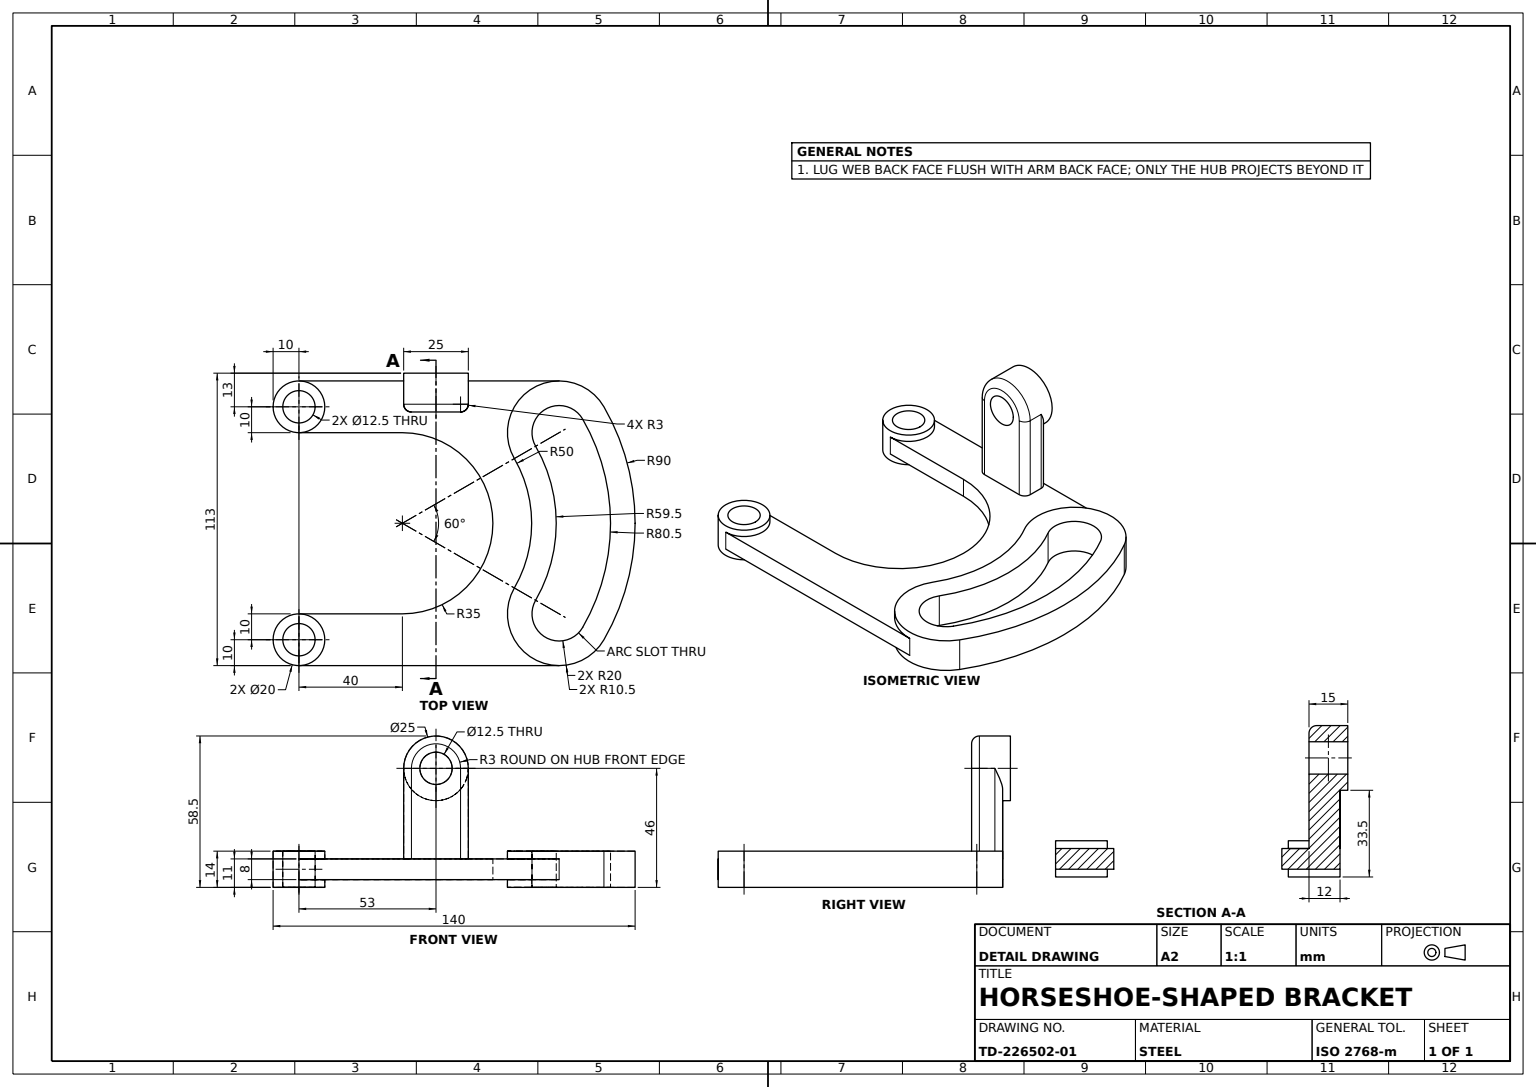
ISO-10303-21;
HEADER;
FILE_DESCRIPTION((''),'2;1');
FILE_NAME('','',(''),(''),'','','');
FILE_SCHEMA(('AUTOMOTIVE_DESIGN'));
ENDSEC;
DATA;
#1=APPLICATION_CONTEXT('');
#2=PRODUCT_CONTEXT('',#1,'mechanical');
#3=PRODUCT('','','',(#2));
#4=PRODUCT_DEFINITION_FORMATION('','',#3);
#5=PRODUCT_DEFINITION_CONTEXT('',#1,'design');
#6=PRODUCT_DEFINITION('','',#4,#5);
#7=PRODUCT_DEFINITION_SHAPE('','',#6);
#8=(LENGTH_UNIT()NAMED_UNIT(*)SI_UNIT(.MILLI.,.METRE.));
#9=(NAMED_UNIT(*)PLANE_ANGLE_UNIT()SI_UNIT($,.RADIAN.));
#10=(NAMED_UNIT(*)SI_UNIT($,.STERADIAN.)SOLID_ANGLE_UNIT());
#11=UNCERTAINTY_MEASURE_WITH_UNIT(LENGTH_MEASURE(1.E-05),#8,'distance_accuracy_value','');
#12=(GEOMETRIC_REPRESENTATION_CONTEXT(3)GLOBAL_UNCERTAINTY_ASSIGNED_CONTEXT((#11))GLOBAL_UNIT_ASSIGNED_CONTEXT((#8,#9,#10))REPRESENTATION_CONTEXT('',''));
#13=CARTESIAN_POINT('',(-43.,39.,-6.75));
#14=VERTEX_POINT('',#13);
#15=CARTESIAN_POINT('',(-58.,39.,-6.75));
#16=VERTEX_POINT('',#15);
#17=CARTESIAN_POINT('',(-25.,39.,-6.75));
#18=DIRECTION('',(-1.,0.,0.));
#19=VECTOR('',#18,1000.);
#20=LINE('',#17,#19);
#21=EDGE_CURVE('',#14,#16,#20,.T.);
#22=ORIENTED_EDGE('',*,*,#21,.T.);
#23=CARTESIAN_POINT('',(-58.,39.,-19.25));
#24=VERTEX_POINT('',#23);
#25=CARTESIAN_POINT('',(-58.,39.,-13.));
#26=DIRECTION('',(0.,0.,1.));
#27=AXIS2_PLACEMENT_3D('',#25,#18,#26);
#28=CIRCLE('',#27,6.25);
#29=EDGE_CURVE('',#16,#24,#28,.T.);
#30=ORIENTED_EDGE('',*,*,#29,.T.);
#31=CARTESIAN_POINT('',(-43.,39.,-19.25));
#32=VERTEX_POINT('',#31);
#33=CARTESIAN_POINT('',(-25.,39.,-19.25));
#34=LINE('',#33,#19);
#35=EDGE_CURVE('',#32,#24,#34,.T.);
#36=ORIENTED_EDGE('',*,*,#35,.F.);
#37=CARTESIAN_POINT('',(-43.,39.,-13.));
#38=AXIS2_PLACEMENT_3D('',#37,#18,#26);
#39=CIRCLE('',#38,6.25);
#40=EDGE_CURVE('',#14,#32,#39,.T.);
#41=ORIENTED_EDGE('',*,*,#40,.F.);
#42=EDGE_LOOP('',(#22,#30,#36,#41));
#43=FACE_OUTER_BOUND('',#42,.T.);
#44=CARTESIAN_POINT('',(-25.,39.,-13.));
#45=AXIS2_PLACEMENT_3D('',#44,#18,#26);
#46=CYLINDRICAL_SURFACE('',#45,6.25);
#47=ADVANCED_FACE('',(#43),#46,.F.);
#48=CARTESIAN_POINT('',(40.25,-7.,-69.715045));
#49=VERTEX_POINT('',#48);
#50=CARTESIAN_POINT('',(0.,-7.,-80.5));
#51=VERTEX_POINT('',#50);
#52=CARTESIAN_POINT('',(0.,-7.,0.));
#53=DIRECTION('',(0.,1.,0.));
#54=AXIS2_PLACEMENT_3D('',#52,#53,#26);
#55=CIRCLE('',#54,80.5);
#56=EDGE_CURVE('',#49,#51,#55,.T.);
#57=ORIENTED_EDGE('',*,*,#56,.T.);
#58=CARTESIAN_POINT('',(-40.25,-7.,-69.715045));
#59=VERTEX_POINT('',#58);
#60=EDGE_CURVE('',#51,#59,#55,.T.);
#61=ORIENTED_EDGE('',*,*,#60,.T.);
#62=CARTESIAN_POINT('',(-29.75,-7.,-51.528512));
#63=VERTEX_POINT('',#62);
#64=CARTESIAN_POINT('',(-35.,-7.,-60.621778));
#65=DIRECTION('',(0.,-1.,0.));
#66=AXIS2_PLACEMENT_3D('',#64,#65,#26);
#67=CIRCLE('',#66,10.5);
#68=EDGE_CURVE('',#63,#59,#67,.T.);
#69=ORIENTED_EDGE('',*,*,#68,.F.);
#70=CARTESIAN_POINT('',(0.,-7.,-59.5));
#71=VERTEX_POINT('',#70);
#72=CIRCLE('',#54,59.5);
#73=EDGE_CURVE('',#71,#63,#72,.T.);
#74=ORIENTED_EDGE('',*,*,#73,.F.);
#75=CARTESIAN_POINT('',(29.75,-7.,-51.528512));
#76=VERTEX_POINT('',#75);
#77=EDGE_CURVE('',#76,#71,#72,.T.);
#78=ORIENTED_EDGE('',*,*,#77,.F.);
#79=CARTESIAN_POINT('',(35.,-7.,-60.621778));
#80=AXIS2_PLACEMENT_3D('',#79,#53,#26);
#81=CIRCLE('',#80,10.5);
#82=EDGE_CURVE('',#76,#49,#81,.T.);
#83=ORIENTED_EDGE('',*,*,#82,.T.);
#84=EDGE_LOOP('',(#57,#61,#69,#74,#78,#83));
#85=FACE_BOUND('',#84,.T.);
#86=CARTESIAN_POINT('',(25.,-7.,-43.30127));
#87=VERTEX_POINT('',#86);
#88=CARTESIAN_POINT('',(0.,-7.,-50.));
#89=VERTEX_POINT('',#88);
#90=CIRCLE('',#54,50.);
#91=EDGE_CURVE('',#87,#89,#90,.T.);
#92=ORIENTED_EDGE('',*,*,#91,.T.);
#93=CARTESIAN_POINT('',(-25.,-7.,-43.30127));
#94=VERTEX_POINT('',#93);
#95=EDGE_CURVE('',#89,#94,#90,.T.);
#96=ORIENTED_EDGE('',*,*,#95,.T.);
#97=CARTESIAN_POINT('',(-45.,-7.,-77.942286));
#98=VERTEX_POINT('',#97);
#99=CIRCLE('',#66,20.);
#100=EDGE_CURVE('',#94,#98,#99,.T.);
#101=ORIENTED_EDGE('',*,*,#100,.T.);
#102=CARTESIAN_POINT('',(0.,-7.,-90.));
#103=VERTEX_POINT('',#102);
#104=CIRCLE('',#54,90.);
#105=EDGE_CURVE('',#103,#98,#104,.T.);
#106=ORIENTED_EDGE('',*,*,#105,.F.);
#107=CARTESIAN_POINT('',(45.,-7.,-77.942286));
#108=VERTEX_POINT('',#107);
#109=EDGE_CURVE('',#108,#103,#104,.T.);
#110=ORIENTED_EDGE('',*,*,#109,.F.);
#111=CIRCLE('',#80,20.);
#112=EDGE_CURVE('',#87,#108,#111,.T.);
#113=ORIENTED_EDGE('',*,*,#112,.F.);
#114=EDGE_LOOP('',(#92,#96,#101,#106,#110,#113));
#115=FACE_OUTER_BOUND('',#114,.T.);
#116=PLANE('',#54);
#117=ADVANCED_FACE('',(#85,#115),#116,.F.);
#118=CARTESIAN_POINT('',(-35.,4.,0.));
#119=VERTEX_POINT('',#118);
#120=CARTESIAN_POINT('',(0.,4.,-35.));
#121=VERTEX_POINT('',#120);
#122=CARTESIAN_POINT('',(0.,4.,0.));
#123=AXIS2_PLACEMENT_3D('',#122,#65,#26);
#124=CIRCLE('',#123,35.);
#125=EDGE_CURVE('',#119,#121,#124,.T.);
#126=ORIENTED_EDGE('',*,*,#125,.F.);
#127=CARTESIAN_POINT('',(-35.,-4.,0.));
#128=VERTEX_POINT('',#127);
#129=VECTOR('',#65,1000.);
#130=LINE('',#118,#129);
#131=EDGE_CURVE('',#119,#128,#130,.T.);
#132=ORIENTED_EDGE('',*,*,#131,.T.);
#133=CARTESIAN_POINT('',(0.,-4.,-35.));
#134=VERTEX_POINT('',#133);
#135=CARTESIAN_POINT('',(0.,-4.,0.));
#136=AXIS2_PLACEMENT_3D('',#135,#65,#26);
#137=CIRCLE('',#136,35.);
#138=EDGE_CURVE('',#128,#134,#137,.T.);
#139=ORIENTED_EDGE('',*,*,#138,.T.);
#140=LINE('',#120,#129);
#141=EDGE_CURVE('',#121,#134,#140,.T.);
#142=ORIENTED_EDGE('',*,*,#141,.F.);
#143=EDGE_LOOP('',(#126,#132,#139,#142));
#144=FACE_OUTER_BOUND('',#143,.T.);
#145=DIRECTION('',(0.,0.,-1.));
#146=AXIS2_PLACEMENT_3D('',#122,#65,#145);
#147=CYLINDRICAL_SURFACE('',#146,35.);
#148=ADVANCED_FACE('',(#144),#147,.F.);
#149=CARTESIAN_POINT('',(-45.,7.,50.));
#150=VERTEX_POINT('',#149);
#151=CARTESIAN_POINT('',(-45.,7.,30.));
#152=VERTEX_POINT('',#151);
#153=CARTESIAN_POINT('',(-45.,7.,40.));
#154=AXIS2_PLACEMENT_3D('',#153,#53,#26);
#155=CIRCLE('',#154,10.);
#156=EDGE_CURVE('',#150,#152,#155,.T.);
#157=ORIENTED_EDGE('',*,*,#156,.T.);
#158=EDGE_CURVE('',#152,#150,#155,.T.);
#159=ORIENTED_EDGE('',*,*,#158,.T.);
#160=EDGE_LOOP('',(#157,#159));
#161=FACE_OUTER_BOUND('',#160,.T.);
#162=CARTESIAN_POINT('',(-45.,7.,33.75));
#163=VERTEX_POINT('',#162);
#164=CARTESIAN_POINT('',(-45.,7.,46.25));
#165=VERTEX_POINT('',#164);
#166=CIRCLE('',#154,6.25);
#167=EDGE_CURVE('',#163,#165,#166,.T.);
#168=ORIENTED_EDGE('',*,*,#167,.F.);
#169=EDGE_CURVE('',#165,#163,#166,.T.);
#170=ORIENTED_EDGE('',*,*,#169,.F.);
#171=EDGE_LOOP('',(#168,#170));
#172=FACE_BOUND('',#171,.T.);
#173=PLANE('',#154);
#174=ADVANCED_FACE('',(#161,#172),#173,.T.);
#175=CARTESIAN_POINT('',(0.,7.,-59.5));
#176=VERTEX_POINT('',#175);
#177=LINE('',#175,#129);
#178=EDGE_CURVE('',#176,#71,#177,.T.);
#179=ORIENTED_EDGE('',*,*,#178,.T.);
#180=ORIENTED_EDGE('',*,*,#73,.T.);
#181=CARTESIAN_POINT('',(-29.75,7.,-51.528512));
#182=VERTEX_POINT('',#181);
#183=LINE('',#181,#129);
#184=EDGE_CURVE('',#182,#63,#183,.T.);
#185=ORIENTED_EDGE('',*,*,#184,.F.);
#186=CARTESIAN_POINT('',(0.,7.,0.));
#187=AXIS2_PLACEMENT_3D('',#186,#53,#26);
#188=CIRCLE('',#187,59.5);
#189=EDGE_CURVE('',#176,#182,#188,.T.);
#190=ORIENTED_EDGE('',*,*,#189,.F.);
#191=EDGE_LOOP('',(#179,#180,#185,#190));
#192=FACE_OUTER_BOUND('',#191,.T.);
#193=AXIS2_PLACEMENT_3D('',#186,#65,#145);
#194=CYLINDRICAL_SURFACE('',#193,59.5);
#195=ADVANCED_FACE('',(#192),#194,.T.);
#196=CARTESIAN_POINT('',(-46.,39.,-25.5));
#197=VERTEX_POINT('',#196);
#198=CARTESIAN_POINT('',(-52.,39.,-25.5));
#199=VERTEX_POINT('',#198);
#200=CARTESIAN_POINT('',(-43.,39.,-25.5));
#201=LINE('',#200,#19);
#202=EDGE_CURVE('',#197,#199,#201,.T.);
#203=ORIENTED_EDGE('',*,*,#202,.T.);
#204=CARTESIAN_POINT('',(-58.,39.,-25.5));
#205=VERTEX_POINT('',#204);
#206=EDGE_CURVE('',#199,#205,#201,.T.);
#207=ORIENTED_EDGE('',*,*,#206,.T.);
#208=CARTESIAN_POINT('',(-58.,39.,-0.5));
#209=VERTEX_POINT('',#208);
#210=CIRCLE('',#27,12.5);
#211=EDGE_CURVE('',#209,#205,#210,.T.);
#212=ORIENTED_EDGE('',*,*,#211,.F.);
#213=CARTESIAN_POINT('',(-52.,39.,-0.5));
#214=VERTEX_POINT('',#213);
#215=CARTESIAN_POINT('',(-43.,39.,-0.5));
#216=LINE('',#215,#19);
#217=EDGE_CURVE('',#214,#209,#216,.T.);
#218=ORIENTED_EDGE('',*,*,#217,.F.);
#219=CARTESIAN_POINT('',(-46.,39.,-0.5));
#220=VERTEX_POINT('',#219);
#221=EDGE_CURVE('',#220,#214,#216,.T.);
#222=ORIENTED_EDGE('',*,*,#221,.F.);
#223=CARTESIAN_POINT('',(-46.,39.,-13.));
#224=AXIS2_PLACEMENT_3D('',#223,#18,#26);
#225=CIRCLE('',#224,12.5);
#226=EDGE_CURVE('',#220,#197,#225,.T.);
#227=ORIENTED_EDGE('',*,*,#226,.T.);
#228=EDGE_LOOP('',(#203,#207,#212,#218,#222,#227));
#229=FACE_OUTER_BOUND('',#228,.T.);
#230=CYLINDRICAL_SURFACE('',#38,12.5);
#231=ADVANCED_FACE('',(#229),#230,.T.);
#232=CARTESIAN_POINT('',(-55.,4.,-3.5));
#233=VERTEX_POINT('',#232);
#234=CARTESIAN_POINT('',(-55.,4.,40.));
#235=VERTEX_POINT('',#234);
#236=CARTESIAN_POINT('',(-55.,4.,-60.621779));
#237=VECTOR('',#26,1000.);
#238=LINE('',#236,#237);
#239=EDGE_CURVE('',#233,#235,#238,.T.);
#240=ORIENTED_EDGE('',*,*,#239,.F.);
#241=CARTESIAN_POINT('',(-55.,30.875962,-3.5));
#242=VERTEX_POINT('',#241);
#243=VECTOR('',#53,1000.);
#244=LINE('',#232,#243);
#245=EDGE_CURVE('',#233,#242,#244,.T.);
#246=ORIENTED_EDGE('',*,*,#245,.T.);
#247=CARTESIAN_POINT('',(-55.,30.875962,-22.5));
#248=VERTEX_POINT('',#247);
#249=CARTESIAN_POINT('',(-55.,39.,-13.));
#250=AXIS2_PLACEMENT_3D('',#249,#18,#26);
#251=CIRCLE('',#250,12.5);
#252=EDGE_CURVE('',#248,#242,#251,.T.);
#253=ORIENTED_EDGE('',*,*,#252,.F.);
#254=CARTESIAN_POINT('',(-55.,4.,-22.5));
#255=VERTEX_POINT('',#254);
#256=LINE('',#254,#129);
#257=EDGE_CURVE('',#248,#255,#256,.T.);
#258=ORIENTED_EDGE('',*,*,#257,.T.);
#259=CARTESIAN_POINT('',(-55.,4.,-60.621778));
#260=VERTEX_POINT('',#259);
#261=EDGE_CURVE('',#260,#255,#238,.T.);
#262=ORIENTED_EDGE('',*,*,#261,.F.);
#263=CARTESIAN_POINT('',(-55.,-4.,-60.621778));
#264=VERTEX_POINT('',#263);
#265=LINE('',#236,#129);
#266=EDGE_CURVE('',#260,#264,#265,.T.);
#267=ORIENTED_EDGE('',*,*,#266,.T.);
#268=CARTESIAN_POINT('',(-55.,-4.,40.));
#269=VERTEX_POINT('',#268);
#270=CARTESIAN_POINT('',(-55.,-4.,-60.621779));
#271=LINE('',#270,#237);
#272=EDGE_CURVE('',#264,#269,#271,.T.);
#273=ORIENTED_EDGE('',*,*,#272,.T.);
#274=LINE('',#234,#129);
#275=EDGE_CURVE('',#235,#269,#274,.T.);
#276=ORIENTED_EDGE('',*,*,#275,.F.);
#277=EDGE_LOOP('',(#240,#246,#253,#258,#262,#267,#273,#276));
#278=FACE_OUTER_BOUND('',#277,.T.);
#279=DIRECTION('',(1.,0.,0.));
#280=AXIS2_PLACEMENT_3D('',#236,#279,#145);
#281=PLANE('',#280);
#282=ADVANCED_FACE('',(#278),#281,.F.);
#283=CARTESIAN_POINT('',(45.,7.,30.));
#284=VERTEX_POINT('',#283);
#285=CARTESIAN_POINT('',(45.,7.,50.));
#286=VERTEX_POINT('',#285);
#287=CARTESIAN_POINT('',(45.,7.,40.));
#288=AXIS2_PLACEMENT_3D('',#287,#53,#26);
#289=CIRCLE('',#288,10.);
#290=EDGE_CURVE('',#284,#286,#289,.T.);
#291=ORIENTED_EDGE('',*,*,#290,.T.);
#292=EDGE_CURVE('',#286,#284,#289,.T.);
#293=ORIENTED_EDGE('',*,*,#292,.T.);
#294=EDGE_LOOP('',(#291,#293));
#295=FACE_OUTER_BOUND('',#294,.T.);
#296=CARTESIAN_POINT('',(45.,7.,33.75));
#297=VERTEX_POINT('',#296);
#298=CARTESIAN_POINT('',(45.,7.,46.25));
#299=VERTEX_POINT('',#298);
#300=CIRCLE('',#288,6.25);
#301=EDGE_CURVE('',#297,#299,#300,.T.);
#302=ORIENTED_EDGE('',*,*,#301,.F.);
#303=EDGE_CURVE('',#299,#297,#300,.T.);
#304=ORIENTED_EDGE('',*,*,#303,.F.);
#305=EDGE_LOOP('',(#302,#304));
#306=FACE_BOUND('',#305,.T.);
#307=PLANE('',#288);
#308=ADVANCED_FACE('',(#295,#306),#307,.T.);
#309=CARTESIAN_POINT('',(0.,-4.,-50.));
#310=VERTEX_POINT('',#309);
#311=CARTESIAN_POINT('',(0.,7.,-50.));
#312=LINE('',#311,#129);
#313=EDGE_CURVE('',#310,#89,#312,.T.);
#314=ORIENTED_EDGE('',*,*,#313,.F.);
#315=CARTESIAN_POINT('',(-25.,-4.,-43.30127));
#316=VERTEX_POINT('',#315);
#317=AXIS2_PLACEMENT_3D('',#135,#53,#26);
#318=CIRCLE('',#317,50.);
#319=EDGE_CURVE('',#310,#316,#318,.T.);
#320=ORIENTED_EDGE('',*,*,#319,.T.);
#321=CARTESIAN_POINT('',(-25.,7.,-43.30127));
#322=LINE('',#321,#129);
#323=EDGE_CURVE('',#316,#94,#322,.T.);
#324=ORIENTED_EDGE('',*,*,#323,.T.);
#325=ORIENTED_EDGE('',*,*,#95,.F.);
#326=EDGE_LOOP('',(#314,#320,#324,#325));
#327=FACE_OUTER_BOUND('',#326,.T.);
#328=CYLINDRICAL_SURFACE('',#193,50.);
#329=ADVANCED_FACE('',(#327),#328,.F.);
#330=CARTESIAN_POINT('',(-45.,-7.,30.));
#331=VERTEX_POINT('',#330);
#332=CARTESIAN_POINT('',(-45.,-7.,50.));
#333=VERTEX_POINT('',#332);
#334=CARTESIAN_POINT('',(-45.,-7.,40.));
#335=AXIS2_PLACEMENT_3D('',#334,#53,#26);
#336=CIRCLE('',#335,10.);
#337=EDGE_CURVE('',#331,#333,#336,.T.);
#338=ORIENTED_EDGE('',*,*,#337,.T.);
#339=LINE('',#332,#243);
#340=EDGE_CURVE('',#333,#150,#339,.T.);
#341=ORIENTED_EDGE('',*,*,#340,.T.);
#342=ORIENTED_EDGE('',*,*,#158,.F.);
#343=CARTESIAN_POINT('',(-45.,4.,30.));
#344=VERTEX_POINT('',#343);
#345=LINE('',#330,#243);
#346=EDGE_CURVE('',#344,#152,#345,.T.);
#347=ORIENTED_EDGE('',*,*,#346,.F.);
#348=CARTESIAN_POINT('',(-45.,4.,40.));
#349=AXIS2_PLACEMENT_3D('',#348,#65,#145);
#350=CIRCLE('',#349,10.);
#351=EDGE_CURVE('',#235,#344,#350,.T.);
#352=ORIENTED_EDGE('',*,*,#351,.F.);
#353=ORIENTED_EDGE('',*,*,#275,.T.);
#354=CARTESIAN_POINT('',(-45.,-4.,30.));
#355=VERTEX_POINT('',#354);
#356=CARTESIAN_POINT('',(-45.,-4.,40.));
#357=AXIS2_PLACEMENT_3D('',#356,#65,#145);
#358=CIRCLE('',#357,10.);
#359=EDGE_CURVE('',#269,#355,#358,.T.);
#360=ORIENTED_EDGE('',*,*,#359,.T.);
#361=EDGE_CURVE('',#331,#355,#345,.T.);
#362=ORIENTED_EDGE('',*,*,#361,.F.);
#363=EDGE_LOOP('',(#338,#341,#342,#347,#352,#353,#360,#362));
#364=FACE_OUTER_BOUND('',#363,.T.);
#365=CYLINDRICAL_SURFACE('',#335,10.);
#366=ADVANCED_FACE('',(#364),#365,.T.);
#367=ORIENTED_EDGE('',*,*,#77,.T.);
#368=ORIENTED_EDGE('',*,*,#178,.F.);
#369=CARTESIAN_POINT('',(29.75,7.,-51.528512));
#370=VERTEX_POINT('',#369);
#371=EDGE_CURVE('',#370,#176,#188,.T.);
#372=ORIENTED_EDGE('',*,*,#371,.F.);
#373=LINE('',#369,#129);
#374=EDGE_CURVE('',#370,#76,#373,.T.);
#375=ORIENTED_EDGE('',*,*,#374,.T.);
#376=EDGE_LOOP('',(#367,#368,#372,#375));
#377=FACE_OUTER_BOUND('',#376,.T.);
#378=ADVANCED_FACE('',(#377),#194,.T.);
#379=CARTESIAN_POINT('',(35.,4.,0.));
#380=VERTEX_POINT('',#379);
#381=CARTESIAN_POINT('',(35.,4.,40.));
#382=VERTEX_POINT('',#381);
#383=LINE('',#379,#237);
#384=EDGE_CURVE('',#380,#382,#383,.T.);
#385=ORIENTED_EDGE('',*,*,#384,.F.);
#386=CARTESIAN_POINT('',(35.,-4.,0.));
#387=VERTEX_POINT('',#386);
#388=LINE('',#379,#129);
#389=EDGE_CURVE('',#380,#387,#388,.T.);
#390=ORIENTED_EDGE('',*,*,#389,.T.);
#391=CARTESIAN_POINT('',(35.,-4.,40.));
#392=VERTEX_POINT('',#391);
#393=LINE('',#386,#237);
#394=EDGE_CURVE('',#387,#392,#393,.T.);
#395=ORIENTED_EDGE('',*,*,#394,.T.);
#396=LINE('',#381,#129);
#397=EDGE_CURVE('',#382,#392,#396,.T.);
#398=ORIENTED_EDGE('',*,*,#397,.F.);
#399=EDGE_LOOP('',(#385,#390,#395,#398));
#400=FACE_OUTER_BOUND('',#399,.T.);
#401=AXIS2_PLACEMENT_3D('',#379,#279,#145);
#402=PLANE('',#401);
#403=ADVANCED_FACE('',(#400),#402,.F.);
#404=CARTESIAN_POINT('',(-35.,-4.,-60.621779));
#405=AXIS2_PLACEMENT_3D('',#404,#65,#26);
#406=CIRCLE('',#405,20.);
#407=EDGE_CURVE('',#316,#264,#406,.T.);
#408=ORIENTED_EDGE('',*,*,#407,.T.);
#409=ORIENTED_EDGE('',*,*,#266,.F.);
#410=CARTESIAN_POINT('',(-25.,4.,-43.30127));
#411=VERTEX_POINT('',#410);
#412=CARTESIAN_POINT('',(-35.,4.,-60.621779));
#413=AXIS2_PLACEMENT_3D('',#412,#65,#26);
#414=CIRCLE('',#413,20.);
#415=EDGE_CURVE('',#411,#260,#414,.T.);
#416=ORIENTED_EDGE('',*,*,#415,.F.);
#417=VERTEX_POINT('',#321);
#418=EDGE_CURVE('',#417,#411,#322,.T.);
#419=ORIENTED_EDGE('',*,*,#418,.F.);
#420=CARTESIAN_POINT('',(-45.,7.,-77.942286));
#421=VERTEX_POINT('',#420);
#422=CARTESIAN_POINT('',(-35.,7.,-60.621778));
#423=AXIS2_PLACEMENT_3D('',#422,#65,#26);
#424=CIRCLE('',#423,20.);
#425=EDGE_CURVE('',#417,#421,#424,.T.);
#426=ORIENTED_EDGE('',*,*,#425,.T.);
#427=LINE('',#420,#129);
#428=EDGE_CURVE('',#421,#98,#427,.T.);
#429=ORIENTED_EDGE('',*,*,#428,.T.);
#430=ORIENTED_EDGE('',*,*,#100,.F.);
#431=ORIENTED_EDGE('',*,*,#323,.F.);
#432=EDGE_LOOP('',(#408,#409,#416,#419,#426,#429,#430,#431));
#433=FACE_OUTER_BOUND('',#432,.T.);
#434=AXIS2_PLACEMENT_3D('',#422,#65,#145);
#435=CYLINDRICAL_SURFACE('',#434,20.);
#436=ADVANCED_FACE('',(#433),#435,.T.);
#437=CARTESIAN_POINT('',(-46.,4.,-25.5));
#438=VERTEX_POINT('',#437);
#439=CARTESIAN_POINT('',(-52.,4.,-25.5));
#440=VERTEX_POINT('',#439);
#441=CARTESIAN_POINT('',(-43.,4.,-25.5));
#442=LINE('',#441,#19);
#443=EDGE_CURVE('',#438,#440,#442,.T.);
#444=ORIENTED_EDGE('',*,*,#443,.T.);
#445=LINE('',#198,#243);
#446=EDGE_CURVE('',#440,#199,#445,.T.);
#447=ORIENTED_EDGE('',*,*,#446,.T.);
#448=ORIENTED_EDGE('',*,*,#202,.F.);
#449=LINE('',#437,#129);
#450=EDGE_CURVE('',#197,#438,#449,.T.);
#451=ORIENTED_EDGE('',*,*,#450,.T.);
#452=EDGE_LOOP('',(#444,#447,#448,#451));
#453=FACE_OUTER_BOUND('',#452,.T.);
#454=CARTESIAN_POINT('',(-43.,0.,-25.5));
#455=AXIS2_PLACEMENT_3D('',#454,#145,#18);
#456=PLANE('',#455);
#457=ADVANCED_FACE('',(#453),#456,.T.);
#458=EDGE_CURVE('',#205,#209,#210,.T.);
#459=ORIENTED_EDGE('',*,*,#458,.T.);
#460=ORIENTED_EDGE('',*,*,#211,.T.);
#461=EDGE_LOOP('',(#459,#460));
#462=FACE_OUTER_BOUND('',#461,.T.);
#463=ORIENTED_EDGE('',*,*,#29,.F.);
#464=EDGE_CURVE('',#24,#16,#28,.T.);
#465=ORIENTED_EDGE('',*,*,#464,.F.);
#466=EDGE_LOOP('',(#463,#465));
#467=FACE_BOUND('',#466,.T.);
#468=PLANE('',#27);
#469=ADVANCED_FACE('',(#462,#467),#468,.T.);
#470=ORIENTED_EDGE('',*,*,#389,.F.);
#471=EDGE_CURVE('',#121,#380,#124,.T.);
#472=ORIENTED_EDGE('',*,*,#471,.F.);
#473=ORIENTED_EDGE('',*,*,#141,.T.);
#474=EDGE_CURVE('',#134,#387,#137,.T.);
#475=ORIENTED_EDGE('',*,*,#474,.T.);
#476=EDGE_LOOP('',(#470,#472,#473,#475));
#477=FACE_OUTER_BOUND('',#476,.T.);
#478=ADVANCED_FACE('',(#477),#147,.F.);
#479=ORIENTED_EDGE('',*,*,#91,.F.);
#480=CARTESIAN_POINT('',(25.,-4.,-43.30127));
#481=VERTEX_POINT('',#480);
#482=CARTESIAN_POINT('',(25.,7.,-43.30127));
#483=LINE('',#482,#129);
#484=EDGE_CURVE('',#481,#87,#483,.T.);
#485=ORIENTED_EDGE('',*,*,#484,.F.);
#486=EDGE_CURVE('',#481,#310,#318,.T.);
#487=ORIENTED_EDGE('',*,*,#486,.T.);
#488=ORIENTED_EDGE('',*,*,#313,.T.);
#489=EDGE_LOOP('',(#479,#485,#487,#488));
#490=FACE_OUTER_BOUND('',#489,.T.);
#491=ADVANCED_FACE('',(#490),#328,.F.);
#492=CARTESIAN_POINT('',(-45.,-7.,46.25));
#493=VERTEX_POINT('',#492);
#494=CARTESIAN_POINT('',(-45.,-38.,46.25));
#495=LINE('',#494,#243);
#496=EDGE_CURVE('',#493,#165,#495,.T.);
#497=ORIENTED_EDGE('',*,*,#496,.T.);
#498=ORIENTED_EDGE('',*,*,#169,.T.);
#499=CARTESIAN_POINT('',(-45.,-7.,33.75));
#500=VERTEX_POINT('',#499);
#501=CARTESIAN_POINT('',(-45.,-38.,33.75));
#502=LINE('',#501,#243);
#503=EDGE_CURVE('',#500,#163,#502,.T.);
#504=ORIENTED_EDGE('',*,*,#503,.F.);
#505=CIRCLE('',#335,6.25);
#506=EDGE_CURVE('',#493,#500,#505,.T.);
#507=ORIENTED_EDGE('',*,*,#506,.F.);
#508=EDGE_LOOP('',(#497,#498,#504,#507));
#509=FACE_OUTER_BOUND('',#508,.T.);
#510=CARTESIAN_POINT('',(-45.,-38.,40.));
#511=AXIS2_PLACEMENT_3D('',#510,#53,#26);
#512=CYLINDRICAL_SURFACE('',#511,6.25);
#513=ADVANCED_FACE('',(#509),#512,.F.);
#514=ORIENTED_EDGE('',*,*,#167,.T.);
#515=ORIENTED_EDGE('',*,*,#496,.F.);
#516=EDGE_CURVE('',#500,#493,#505,.T.);
#517=ORIENTED_EDGE('',*,*,#516,.F.);
#518=ORIENTED_EDGE('',*,*,#503,.T.);
#519=EDGE_LOOP('',(#514,#515,#517,#518));
#520=FACE_OUTER_BOUND('',#519,.T.);
#521=ADVANCED_FACE('',(#520),#512,.F.);
#522=EDGE_CURVE('',#32,#14,#39,.T.);
#523=ORIENTED_EDGE('',*,*,#522,.F.);
#524=ORIENTED_EDGE('',*,*,#35,.T.);
#525=ORIENTED_EDGE('',*,*,#464,.T.);
#526=ORIENTED_EDGE('',*,*,#21,.F.);
#527=EDGE_LOOP('',(#523,#524,#525,#526));
#528=FACE_OUTER_BOUND('',#527,.T.);
#529=ADVANCED_FACE('',(#528),#46,.F.);
#530=CARTESIAN_POINT('',(-43.,39.,-22.5));
#531=VERTEX_POINT('',#530);
#532=CARTESIAN_POINT('',(-46.,39.,-22.5));
#533=AXIS2_PLACEMENT_3D('',#532,#65,#145);
#534=CIRCLE('',#533,3.);
#535=EDGE_CURVE('',#197,#531,#534,.T.);
#536=ORIENTED_EDGE('',*,*,#535,.F.);
#537=ORIENTED_EDGE('',*,*,#226,.F.);
#538=CARTESIAN_POINT('',(-43.,39.,-3.5));
#539=VERTEX_POINT('',#538);
#540=CARTESIAN_POINT('',(-46.,39.,-3.5));
#541=AXIS2_PLACEMENT_3D('',#540,#53,#26);
#542=CIRCLE('',#541,3.);
#543=EDGE_CURVE('',#220,#539,#542,.T.);
#544=ORIENTED_EDGE('',*,*,#543,.T.);
#545=AXIS2_PLACEMENT_3D('',#37,#279,#26);
#546=CIRCLE('',#545,9.5);
#547=EDGE_CURVE('',#531,#539,#546,.T.);
#548=ORIENTED_EDGE('',*,*,#547,.F.);
#549=EDGE_LOOP('',(#536,#537,#544,#548));
#550=FACE_OUTER_BOUND('',#549,.T.);
#551=TOROIDAL_SURFACE('',#224,9.5,3.);
#552=ADVANCED_FACE('',(#550),#551,.T.);
#553=CARTESIAN_POINT('',(55.,-4.,40.));
#554=VERTEX_POINT('',#553);
#555=CARTESIAN_POINT('',(55.,-4.,-60.621779));
#556=VERTEX_POINT('',#555);
#557=VECTOR('',#145,1000.);
#558=LINE('',#555,#557);
#559=EDGE_CURVE('',#554,#556,#558,.T.);
#560=ORIENTED_EDGE('',*,*,#559,.T.);
#561=CARTESIAN_POINT('',(55.,4.,-60.621778));
#562=VERTEX_POINT('',#561);
#563=CARTESIAN_POINT('',(55.,4.,-60.621779));
#564=LINE('',#563,#129);
#565=EDGE_CURVE('',#562,#556,#564,.T.);
#566=ORIENTED_EDGE('',*,*,#565,.F.);
#567=CARTESIAN_POINT('',(55.,4.,40.));
#568=VERTEX_POINT('',#567);
#569=LINE('',#567,#557);
#570=EDGE_CURVE('',#568,#562,#569,.T.);
#571=ORIENTED_EDGE('',*,*,#570,.F.);
#572=LINE('',#567,#129);
#573=EDGE_CURVE('',#568,#554,#572,.T.);
#574=ORIENTED_EDGE('',*,*,#573,.T.);
#575=EDGE_LOOP('',(#560,#566,#571,#574));
#576=FACE_OUTER_BOUND('',#575,.T.);
#577=AXIS2_PLACEMENT_3D('',#563,#18,#26);
#578=PLANE('',#577);
#579=ADVANCED_FACE('',(#576),#578,.F.);
#580=ORIENTED_EDGE('',*,*,#397,.T.);
#581=CARTESIAN_POINT('',(45.,-4.,30.));
#582=VERTEX_POINT('',#581);
#583=CARTESIAN_POINT('',(45.,-4.,40.));
#584=AXIS2_PLACEMENT_3D('',#583,#65,#145);
#585=CIRCLE('',#584,10.);
#586=EDGE_CURVE('',#392,#582,#585,.T.);
#587=ORIENTED_EDGE('',*,*,#586,.T.);
#588=CARTESIAN_POINT('',(45.,-7.,30.));
#589=VERTEX_POINT('',#588);
#590=LINE('',#588,#243);
#591=EDGE_CURVE('',#589,#582,#590,.T.);
#592=ORIENTED_EDGE('',*,*,#591,.F.);
#593=CARTESIAN_POINT('',(45.,-7.,50.));
#594=VERTEX_POINT('',#593);
#595=CARTESIAN_POINT('',(45.,-7.,40.));
#596=AXIS2_PLACEMENT_3D('',#595,#53,#26);
#597=CIRCLE('',#596,10.);
#598=EDGE_CURVE('',#589,#594,#597,.T.);
#599=ORIENTED_EDGE('',*,*,#598,.T.);
#600=LINE('',#593,#243);
#601=EDGE_CURVE('',#594,#286,#600,.T.);
#602=ORIENTED_EDGE('',*,*,#601,.T.);
#603=ORIENTED_EDGE('',*,*,#290,.F.);
#604=CARTESIAN_POINT('',(45.,4.,30.));
#605=VERTEX_POINT('',#604);
#606=EDGE_CURVE('',#605,#284,#590,.T.);
#607=ORIENTED_EDGE('',*,*,#606,.F.);
#608=CARTESIAN_POINT('',(45.,4.,40.));
#609=AXIS2_PLACEMENT_3D('',#608,#65,#145);
#610=CIRCLE('',#609,10.);
#611=EDGE_CURVE('',#382,#605,#610,.T.);
#612=ORIENTED_EDGE('',*,*,#611,.F.);
#613=EDGE_LOOP('',(#580,#587,#592,#599,#602,#603,#607,#612));
#614=FACE_OUTER_BOUND('',#613,.T.);
#615=CYLINDRICAL_SURFACE('',#596,10.);
#616=ADVANCED_FACE('',(#614),#615,.T.);
#617=CARTESIAN_POINT('',(25.,4.,-43.30127));
#618=VERTEX_POINT('',#617);
#619=CARTESIAN_POINT('',(0.,4.,-50.));
#620=VERTEX_POINT('',#619);
#621=AXIS2_PLACEMENT_3D('',#122,#53,#26);
#622=CIRCLE('',#621,50.);
#623=EDGE_CURVE('',#618,#620,#622,.T.);
#624=ORIENTED_EDGE('',*,*,#623,.T.);
#625=EDGE_CURVE('',#620,#411,#622,.T.);
#626=ORIENTED_EDGE('',*,*,#625,.T.);
#627=ORIENTED_EDGE('',*,*,#415,.T.);
#628=ORIENTED_EDGE('',*,*,#261,.T.);
#629=CARTESIAN_POINT('',(-52.,4.,-22.5));
#630=AXIS2_PLACEMENT_3D('',#629,#65,#145);
#631=CIRCLE('',#630,3.);
#632=EDGE_CURVE('',#255,#440,#631,.T.);
#633=ORIENTED_EDGE('',*,*,#632,.T.);
#634=ORIENTED_EDGE('',*,*,#443,.F.);
#635=CARTESIAN_POINT('',(-43.,4.,-22.5));
#636=VERTEX_POINT('',#635);
#637=CARTESIAN_POINT('',(-46.,4.,-22.5));
#638=AXIS2_PLACEMENT_3D('',#637,#65,#145);
#639=CIRCLE('',#638,3.);
#640=EDGE_CURVE('',#438,#636,#639,.T.);
#641=ORIENTED_EDGE('',*,*,#640,.T.);
#642=CARTESIAN_POINT('',(-43.,4.,-3.5));
#643=VERTEX_POINT('',#642);
#644=CARTESIAN_POINT('',(-43.,4.,0.));
#645=LINE('',#644,#557);
#646=EDGE_CURVE('',#643,#636,#645,.T.);
#647=ORIENTED_EDGE('',*,*,#646,.F.);
#648=CARTESIAN_POINT('',(-46.,4.,-0.5));
#649=VERTEX_POINT('',#648);
#650=CARTESIAN_POINT('',(-46.,4.,-3.5));
#651=AXIS2_PLACEMENT_3D('',#650,#65,#145);
#652=CIRCLE('',#651,3.);
#653=EDGE_CURVE('',#643,#649,#652,.T.);
#654=ORIENTED_EDGE('',*,*,#653,.T.);
#655=CARTESIAN_POINT('',(-52.,4.,-0.5));
#656=VERTEX_POINT('',#655);
#657=CARTESIAN_POINT('',(-43.,4.,-0.5));
#658=LINE('',#657,#19);
#659=EDGE_CURVE('',#649,#656,#658,.T.);
#660=ORIENTED_EDGE('',*,*,#659,.T.);
#661=CARTESIAN_POINT('',(-52.,4.,-3.5));
#662=AXIS2_PLACEMENT_3D('',#661,#65,#145);
#663=CIRCLE('',#662,3.);
#664=EDGE_CURVE('',#656,#233,#663,.T.);
#665=ORIENTED_EDGE('',*,*,#664,.T.);
#666=ORIENTED_EDGE('',*,*,#239,.T.);
#667=ORIENTED_EDGE('',*,*,#351,.T.);
#668=CARTESIAN_POINT('',(-35.,4.,40.));
#669=VERTEX_POINT('',#668);
#670=EDGE_CURVE('',#344,#669,#350,.T.);
#671=ORIENTED_EDGE('',*,*,#670,.T.);
#672=LINE('',#118,#557);
#673=EDGE_CURVE('',#669,#119,#672,.T.);
#674=ORIENTED_EDGE('',*,*,#673,.T.);
#675=ORIENTED_EDGE('',*,*,#125,.T.);
#676=ORIENTED_EDGE('',*,*,#471,.T.);
#677=ORIENTED_EDGE('',*,*,#384,.T.);
#678=ORIENTED_EDGE('',*,*,#611,.T.);
#679=EDGE_CURVE('',#605,#568,#610,.T.);
#680=ORIENTED_EDGE('',*,*,#679,.T.);
#681=ORIENTED_EDGE('',*,*,#570,.T.);
#682=CARTESIAN_POINT('',(35.,4.,-60.621779));
#683=AXIS2_PLACEMENT_3D('',#682,#65,#145);
#684=CIRCLE('',#683,20.);
#685=EDGE_CURVE('',#562,#618,#684,.T.);
#686=ORIENTED_EDGE('',*,*,#685,.T.);
#687=EDGE_LOOP('',(#624,#626,#627,#628,#633,#634,#641,#647,#654,#660,#665,#666,#667,#671,#674,#675,#676,#677,#678,#680,#681,#686));
#688=FACE_OUTER_BOUND('',#687,.T.);
#689=PLANE('',#683);
#690=ADVANCED_FACE('',(#688),#689,.F.);
#691=CARTESIAN_POINT('',(40.25,7.,-69.715045));
#692=VERTEX_POINT('',#691);
#693=CARTESIAN_POINT('',(35.,7.,-60.621778));
#694=AXIS2_PLACEMENT_3D('',#693,#53,#26);
#695=CIRCLE('',#694,10.5);
#696=EDGE_CURVE('',#370,#692,#695,.T.);
#697=ORIENTED_EDGE('',*,*,#696,.T.);
#698=LINE('',#691,#129);
#699=EDGE_CURVE('',#692,#49,#698,.T.);
#700=ORIENTED_EDGE('',*,*,#699,.T.);
#701=ORIENTED_EDGE('',*,*,#82,.F.);
#702=ORIENTED_EDGE('',*,*,#374,.F.);
#703=EDGE_LOOP('',(#697,#700,#701,#702));
#704=FACE_OUTER_BOUND('',#703,.T.);
#705=AXIS2_PLACEMENT_3D('',#693,#65,#145);
#706=CYLINDRICAL_SURFACE('',#705,10.5);
#707=ADVANCED_FACE('',(#704),#706,.F.);
#708=CARTESIAN_POINT('',(0.,7.,-80.5));
#709=VERTEX_POINT('',#708);
#710=LINE('',#708,#129);
#711=EDGE_CURVE('',#709,#51,#710,.T.);
#712=ORIENTED_EDGE('',*,*,#711,.F.);
#713=CARTESIAN_POINT('',(-40.25,7.,-69.715045));
#714=VERTEX_POINT('',#713);
#715=CIRCLE('',#187,80.5);
#716=EDGE_CURVE('',#709,#714,#715,.T.);
#717=ORIENTED_EDGE('',*,*,#716,.T.);
#718=LINE('',#713,#129);
#719=EDGE_CURVE('',#714,#59,#718,.T.);
#720=ORIENTED_EDGE('',*,*,#719,.T.);
#721=ORIENTED_EDGE('',*,*,#60,.F.);
#722=EDGE_LOOP('',(#712,#717,#720,#721));
#723=FACE_OUTER_BOUND('',#722,.T.);
#724=CYLINDRICAL_SURFACE('',#193,80.5);
#725=ADVANCED_FACE('',(#723),#724,.F.);
#726=ORIENTED_EDGE('',*,*,#105,.T.);
#727=ORIENTED_EDGE('',*,*,#428,.F.);
#728=CARTESIAN_POINT('',(0.,7.,-90.));
#729=VERTEX_POINT('',#728);
#730=CIRCLE('',#187,90.);
#731=EDGE_CURVE('',#729,#421,#730,.T.);
#732=ORIENTED_EDGE('',*,*,#731,.F.);
#733=LINE('',#728,#129);
#734=EDGE_CURVE('',#729,#103,#733,.T.);
#735=ORIENTED_EDGE('',*,*,#734,.T.);
#736=EDGE_LOOP('',(#726,#727,#732,#735));
#737=FACE_OUTER_BOUND('',#736,.T.);
#738=CYLINDRICAL_SURFACE('',#193,90.);
#739=ADVANCED_FACE('',(#737),#738,.T.);
#740=ORIENTED_EDGE('',*,*,#659,.F.);
#741=CARTESIAN_POINT('',(-46.,0.,-0.5));
#742=LINE('',#741,#243);
#743=EDGE_CURVE('',#649,#220,#742,.T.);
#744=ORIENTED_EDGE('',*,*,#743,.T.);
#745=ORIENTED_EDGE('',*,*,#221,.T.);
#746=CARTESIAN_POINT('',(-52.,0.,-0.5));
#747=LINE('',#746,#129);
#748=EDGE_CURVE('',#214,#656,#747,.T.);
#749=ORIENTED_EDGE('',*,*,#748,.T.);
#750=EDGE_LOOP('',(#740,#744,#745,#749));
#751=FACE_OUTER_BOUND('',#750,.T.);
#752=CARTESIAN_POINT('',(-43.,0.,-0.5));
#753=AXIS2_PLACEMENT_3D('',#752,#145,#18);
#754=PLANE('',#753);
#755=ADVANCED_FACE('',(#751),#754,.F.);
#756=EDGE_CURVE('',#333,#331,#336,.T.);
#757=ORIENTED_EDGE('',*,*,#756,.F.);
#758=ORIENTED_EDGE('',*,*,#337,.F.);
#759=EDGE_LOOP('',(#757,#758));
#760=FACE_OUTER_BOUND('',#759,.T.);
#761=ORIENTED_EDGE('',*,*,#506,.T.);
#762=ORIENTED_EDGE('',*,*,#516,.T.);
#763=EDGE_LOOP('',(#761,#762));
#764=FACE_BOUND('',#763,.T.);
#765=PLANE('',#335);
#766=ADVANCED_FACE('',(#760,#764),#765,.F.);
#767=ORIENTED_EDGE('',*,*,#586,.F.);
#768=ORIENTED_EDGE('',*,*,#394,.F.);
#769=ORIENTED_EDGE('',*,*,#474,.F.);
#770=ORIENTED_EDGE('',*,*,#138,.F.);
#771=CARTESIAN_POINT('',(-35.,-4.,40.));
#772=VERTEX_POINT('',#771);
#773=LINE('',#127,#557);
#774=EDGE_CURVE('',#772,#128,#773,.T.);
#775=ORIENTED_EDGE('',*,*,#774,.F.);
#776=EDGE_CURVE('',#355,#772,#358,.T.);
#777=ORIENTED_EDGE('',*,*,#776,.F.);
#778=ORIENTED_EDGE('',*,*,#359,.F.);
#779=ORIENTED_EDGE('',*,*,#272,.F.);
#780=ORIENTED_EDGE('',*,*,#407,.F.);
#781=ORIENTED_EDGE('',*,*,#319,.F.);
#782=ORIENTED_EDGE('',*,*,#486,.F.);
#783=CARTESIAN_POINT('',(35.,-4.,-60.621779));
#784=AXIS2_PLACEMENT_3D('',#783,#65,#145);
#785=CIRCLE('',#784,20.);
#786=EDGE_CURVE('',#556,#481,#785,.T.);
#787=ORIENTED_EDGE('',*,*,#786,.F.);
#788=ORIENTED_EDGE('',*,*,#559,.F.);
#789=EDGE_CURVE('',#582,#554,#585,.T.);
#790=ORIENTED_EDGE('',*,*,#789,.F.);
#791=EDGE_LOOP('',(#767,#768,#769,#770,#775,#777,#778,#779,#780,#781,#782,#787,#788,#790));
#792=FACE_OUTER_BOUND('',#791,.T.);
#793=PLANE('',#784);
#794=ADVANCED_FACE('',(#792),#793,.T.);
#795=ORIENTED_EDGE('',*,*,#748,.F.);
#796=CARTESIAN_POINT('',(-55.,31.177664,-3.241996));
#797=CARTESIAN_POINT('',(-54.967361,31.486776,-3.002418));
#798=CARTESIAN_POINT('',(-54.856939,32.120492,-2.55622));
#799=CARTESIAN_POINT('',(-54.77889,32.445081,-2.349641));
#800=CARTESIAN_POINT('',(-54.492612,33.443005,-1.776889));
#801=CARTESIAN_POINT('',(-54.240564,34.117086,-1.470231));
#802=CARTESIAN_POINT('',(-53.815015,35.14414,-1.104015));
#803=CARTESIAN_POINT('',(-53.664734,35.489382,-0.997691));
#804=CARTESIAN_POINT('',(-53.351167,36.1867,-0.81537));
#805=CARTESIAN_POINT('',(-53.18808,36.538234,-0.739648));
#806=CARTESIAN_POINT('',(-52.856617,37.239397,-0.619499));
#807=CARTESIAN_POINT('',(-52.687681,37.590243,-0.574737));
#808=CARTESIAN_POINT('',(-52.431457,38.117786,-0.529922));
#809=CARTESIAN_POINT('',(-52.345574,38.293845,-0.518714));
#810=CARTESIAN_POINT('',(-52.173164,38.64653,-0.503752));
#811=CARTESIAN_POINT('',(-52.086103,38.824242,-0.5));
#812=B_SPLINE_CURVE_WITH_KNOTS('',3,(#241,#796,#797,#798,#799,#800,#801,#802,#803,#804,#805,#806,#807,#808,#809,#810,#811,#213),.UNSPECIFIED.,.F.,.F.,(4,2,2,2,2,2,2,2,4),(0.,0.001174292,0.002348585,0.00469717,0.005871462,0.007045754,0.008220047,0.008807193,0.009394339),.UNSPECIFIED.);
#813=EDGE_CURVE('',#242,#214,#812,.T.);
#814=ORIENTED_EDGE('',*,*,#813,.F.);
#815=ORIENTED_EDGE('',*,*,#245,.F.);
#816=ORIENTED_EDGE('',*,*,#664,.F.);
#817=EDGE_LOOP('',(#795,#814,#815,#816));
#818=FACE_OUTER_BOUND('',#817,.T.);
#819=CARTESIAN_POINT('',(-52.,0.,-3.5));
#820=AXIS2_PLACEMENT_3D('',#819,#65,#145);
#821=CYLINDRICAL_SURFACE('',#820,3.);
#822=ADVANCED_FACE('',(#818),#821,.T.);
#823=EDGE_CURVE('',#692,#709,#715,.T.);
#824=ORIENTED_EDGE('',*,*,#823,.T.);
#825=ORIENTED_EDGE('',*,*,#711,.T.);
#826=ORIENTED_EDGE('',*,*,#56,.F.);
#827=ORIENTED_EDGE('',*,*,#699,.F.);
#828=EDGE_LOOP('',(#824,#825,#826,#827));
#829=FACE_OUTER_BOUND('',#828,.T.);
#830=ADVANCED_FACE('',(#829),#724,.F.);
#831=ORIENTED_EDGE('',*,*,#450,.F.);
#832=ORIENTED_EDGE('',*,*,#535,.T.);
#833=LINE('',#530,#243);
#834=EDGE_CURVE('',#636,#531,#833,.T.);
#835=ORIENTED_EDGE('',*,*,#834,.F.);
#836=ORIENTED_EDGE('',*,*,#640,.F.);
#837=EDGE_LOOP('',(#831,#832,#835,#836));
#838=FACE_OUTER_BOUND('',#837,.T.);
#839=CARTESIAN_POINT('',(-46.,0.,-22.5));
#840=AXIS2_PLACEMENT_3D('',#839,#53,#26);
#841=CYLINDRICAL_SURFACE('',#840,3.);
#842=ADVANCED_FACE('',(#838),#841,.T.);
#843=ORIENTED_EDGE('',*,*,#301,.T.);
#844=CARTESIAN_POINT('',(45.,-7.,46.25));
#845=VERTEX_POINT('',#844);
#846=CARTESIAN_POINT('',(45.,-38.,46.25));
#847=LINE('',#846,#243);
#848=EDGE_CURVE('',#845,#299,#847,.T.);
#849=ORIENTED_EDGE('',*,*,#848,.F.);
#850=CARTESIAN_POINT('',(45.,-7.,33.75));
#851=VERTEX_POINT('',#850);
#852=CIRCLE('',#596,6.25);
#853=EDGE_CURVE('',#851,#845,#852,.T.);
#854=ORIENTED_EDGE('',*,*,#853,.F.);
#855=CARTESIAN_POINT('',(45.,-38.,33.75));
#856=LINE('',#855,#243);
#857=EDGE_CURVE('',#851,#297,#856,.T.);
#858=ORIENTED_EDGE('',*,*,#857,.T.);
#859=EDGE_LOOP('',(#843,#849,#854,#858));
#860=FACE_OUTER_BOUND('',#859,.T.);
#861=CARTESIAN_POINT('',(45.,-38.,40.));
#862=AXIS2_PLACEMENT_3D('',#861,#53,#26);
#863=CYLINDRICAL_SURFACE('',#862,6.25);
#864=ADVANCED_FACE('',(#860),#863,.F.);
#865=ORIENTED_EDGE('',*,*,#601,.F.);
#866=EDGE_CURVE('',#594,#589,#597,.T.);
#867=ORIENTED_EDGE('',*,*,#866,.T.);
#868=ORIENTED_EDGE('',*,*,#591,.T.);
#869=ORIENTED_EDGE('',*,*,#789,.T.);
#870=ORIENTED_EDGE('',*,*,#573,.F.);
#871=ORIENTED_EDGE('',*,*,#679,.F.);
#872=ORIENTED_EDGE('',*,*,#606,.T.);
#873=ORIENTED_EDGE('',*,*,#292,.F.);
#874=EDGE_LOOP('',(#865,#867,#868,#869,#870,#871,#872,#873));
#875=FACE_OUTER_BOUND('',#874,.T.);
#876=ADVANCED_FACE('',(#875),#615,.T.);
#877=ORIENTED_EDGE('',*,*,#547,.T.);
#878=CARTESIAN_POINT('',(-43.,0.,-3.5));
#879=LINE('',#878,#129);
#880=EDGE_CURVE('',#539,#643,#879,.T.);
#881=ORIENTED_EDGE('',*,*,#880,.T.);
#882=ORIENTED_EDGE('',*,*,#646,.T.);
#883=ORIENTED_EDGE('',*,*,#834,.T.);
#884=EDGE_LOOP('',(#877,#881,#882,#883));
#885=FACE_OUTER_BOUND('',#884,.T.);
#886=ORIENTED_EDGE('',*,*,#40,.T.);
#887=ORIENTED_EDGE('',*,*,#522,.T.);
#888=EDGE_LOOP('',(#886,#887));
#889=FACE_BOUND('',#888,.T.);
#890=CARTESIAN_POINT('',(-43.,0.,0.));
#891=AXIS2_PLACEMENT_3D('',#890,#18,#26);
#892=PLANE('',#891);
#893=ADVANCED_FACE('',(#885,#889),#892,.F.);
#894=ORIENTED_EDGE('',*,*,#632,.F.);
#895=ORIENTED_EDGE('',*,*,#257,.F.);
#896=CARTESIAN_POINT('',(-52.172434,38.648021,-25.5));
#897=CARTESIAN_POINT('',(-52.34606,38.293609,-25.485015));
#898=CARTESIAN_POINT('',(-52.687692,37.590221,-25.425261));
#899=CARTESIAN_POINT('',(-52.856627,37.239376,-25.380497));
#900=CARTESIAN_POINT('',(-53.188089,36.538215,-25.260348));
#901=CARTESIAN_POINT('',(-53.351175,36.186682,-25.184626));
#902=CARTESIAN_POINT('',(-53.664741,35.489366,-25.002305));
#903=CARTESIAN_POINT('',(-53.815021,35.144126,-24.89598));
#904=CARTESIAN_POINT('',(-54.240568,34.117076,-24.529765));
#905=CARTESIAN_POINT('',(-54.492614,33.442997,-24.223106));
#906=CARTESIAN_POINT('',(-54.778891,32.445076,-23.650355));
#907=CARTESIAN_POINT('',(-54.85694,32.120488,-23.443777));
#908=CARTESIAN_POINT('',(-54.967362,31.486774,-22.99758));
#909=CARTESIAN_POINT('',(-55.,31.177663,-22.758004));
#910=B_SPLINE_CURVE_WITH_KNOTS('',3,(#198,#896,#897,#898,#899,#900,#901,#902,#903,#904,#905,#906,#907,#908,#909,#247),.UNSPECIFIED.,.F.,.F.,(4,2,2,2,2,2,2,4),(-0.000022361,0.001153481,0.002329323,0.003505164,0.004681006,0.00703269,0.008208531,0.009384373),.UNSPECIFIED.);
#911=EDGE_CURVE('',#199,#248,#910,.T.);
#912=ORIENTED_EDGE('',*,*,#911,.F.);
#913=ORIENTED_EDGE('',*,*,#446,.F.);
#914=EDGE_LOOP('',(#894,#895,#912,#913));
#915=FACE_OUTER_BOUND('',#914,.T.);
#916=AXIS2_PLACEMENT_3D('',#629,#53,#26);
#917=CYLINDRICAL_SURFACE('',#916,3.);
#918=ADVANCED_FACE('',(#915),#917,.T.);
#919=ORIENTED_EDGE('',*,*,#418,.T.);
#920=ORIENTED_EDGE('',*,*,#625,.F.);
#921=VERTEX_POINT('',#311);
#922=EDGE_CURVE('',#921,#620,#312,.T.);
#923=ORIENTED_EDGE('',*,*,#922,.F.);
#924=CIRCLE('',#187,50.);
#925=EDGE_CURVE('',#921,#417,#924,.T.);
#926=ORIENTED_EDGE('',*,*,#925,.T.);
#927=EDGE_LOOP('',(#919,#920,#923,#926));
#928=FACE_OUTER_BOUND('',#927,.T.);
#929=ADVANCED_FACE('',(#928),#328,.F.);
#930=LINE('',#668,#129);
#931=EDGE_CURVE('',#669,#772,#930,.T.);
#932=ORIENTED_EDGE('',*,*,#931,.F.);
#933=ORIENTED_EDGE('',*,*,#670,.F.);
#934=ORIENTED_EDGE('',*,*,#346,.T.);
#935=ORIENTED_EDGE('',*,*,#156,.F.);
#936=ORIENTED_EDGE('',*,*,#340,.F.);
#937=ORIENTED_EDGE('',*,*,#756,.T.);
#938=ORIENTED_EDGE('',*,*,#361,.T.);
#939=ORIENTED_EDGE('',*,*,#776,.T.);
#940=EDGE_LOOP('',(#932,#933,#934,#935,#936,#937,#938,#939));
#941=FACE_OUTER_BOUND('',#940,.T.);
#942=ADVANCED_FACE('',(#941),#365,.T.);
#943=CIRCLE('',#423,10.5);
#944=EDGE_CURVE('',#182,#714,#943,.T.);
#945=ORIENTED_EDGE('',*,*,#944,.F.);
#946=ORIENTED_EDGE('',*,*,#184,.T.);
#947=ORIENTED_EDGE('',*,*,#68,.T.);
#948=ORIENTED_EDGE('',*,*,#719,.F.);
#949=EDGE_LOOP('',(#945,#946,#947,#948));
#950=FACE_OUTER_BOUND('',#949,.T.);
#951=CYLINDRICAL_SURFACE('',#434,10.5);
#952=ADVANCED_FACE('',(#950),#951,.F.);
#953=ORIENTED_EDGE('',*,*,#371,.T.);
#954=ORIENTED_EDGE('',*,*,#189,.T.);
#955=ORIENTED_EDGE('',*,*,#944,.T.);
#956=ORIENTED_EDGE('',*,*,#716,.F.);
#957=ORIENTED_EDGE('',*,*,#823,.F.);
#958=ORIENTED_EDGE('',*,*,#696,.F.);
#959=EDGE_LOOP('',(#953,#954,#955,#956,#957,#958));
#960=FACE_BOUND('',#959,.T.);
#961=ORIENTED_EDGE('',*,*,#425,.F.);
#962=ORIENTED_EDGE('',*,*,#925,.F.);
#963=VERTEX_POINT('',#482);
#964=EDGE_CURVE('',#963,#921,#924,.T.);
#965=ORIENTED_EDGE('',*,*,#964,.F.);
#966=CARTESIAN_POINT('',(45.,7.,-77.942286));
#967=VERTEX_POINT('',#966);
#968=CIRCLE('',#694,20.);
#969=EDGE_CURVE('',#963,#967,#968,.T.);
#970=ORIENTED_EDGE('',*,*,#969,.T.);
#971=EDGE_CURVE('',#967,#729,#730,.T.);
#972=ORIENTED_EDGE('',*,*,#971,.T.);
#973=ORIENTED_EDGE('',*,*,#731,.T.);
#974=EDGE_LOOP('',(#961,#962,#965,#970,#972,#973));
#975=FACE_OUTER_BOUND('',#974,.T.);
#976=PLANE('',#187);
#977=ADVANCED_FACE('',(#960,#975),#976,.T.);
#978=ORIENTED_EDGE('',*,*,#853,.T.);
#979=EDGE_CURVE('',#845,#851,#852,.T.);
#980=ORIENTED_EDGE('',*,*,#979,.T.);
#981=EDGE_LOOP('',(#978,#980));
#982=FACE_BOUND('',#981,.T.);
#983=ORIENTED_EDGE('',*,*,#598,.F.);
#984=ORIENTED_EDGE('',*,*,#866,.F.);
#985=EDGE_LOOP('',(#983,#984));
#986=FACE_OUTER_BOUND('',#985,.T.);
#987=PLANE('',#596);
#988=ADVANCED_FACE('',(#982,#986),#987,.F.);
#989=ORIENTED_EDGE('',*,*,#848,.T.);
#990=ORIENTED_EDGE('',*,*,#303,.T.);
#991=ORIENTED_EDGE('',*,*,#857,.F.);
#992=ORIENTED_EDGE('',*,*,#979,.F.);
#993=EDGE_LOOP('',(#989,#990,#991,#992));
#994=FACE_OUTER_BOUND('',#993,.T.);
#995=ADVANCED_FACE('',(#994),#863,.F.);
#996=ORIENTED_EDGE('',*,*,#623,.F.);
#997=EDGE_CURVE('',#963,#618,#483,.T.);
#998=ORIENTED_EDGE('',*,*,#997,.F.);
#999=ORIENTED_EDGE('',*,*,#964,.T.);
#1000=ORIENTED_EDGE('',*,*,#922,.T.);
#1001=EDGE_LOOP('',(#996,#998,#999,#1000));
#1002=FACE_OUTER_BOUND('',#1001,.T.);
#1003=ADVANCED_FACE('',(#1002),#328,.F.);
#1004=ORIENTED_EDGE('',*,*,#673,.F.);
#1005=ORIENTED_EDGE('',*,*,#931,.T.);
#1006=ORIENTED_EDGE('',*,*,#774,.T.);
#1007=ORIENTED_EDGE('',*,*,#131,.F.);
#1008=EDGE_LOOP('',(#1004,#1005,#1006,#1007));
#1009=FACE_OUTER_BOUND('',#1008,.T.);
#1010=AXIS2_PLACEMENT_3D('',#118,#18,#26);
#1011=PLANE('',#1010);
#1012=ADVANCED_FACE('',(#1009),#1011,.F.);
#1013=ORIENTED_EDGE('',*,*,#743,.F.);
#1014=ORIENTED_EDGE('',*,*,#653,.F.);
#1015=ORIENTED_EDGE('',*,*,#880,.F.);
#1016=ORIENTED_EDGE('',*,*,#543,.F.);
#1017=EDGE_LOOP('',(#1013,#1014,#1015,#1016));
#1018=FACE_OUTER_BOUND('',#1017,.T.);
#1019=CARTESIAN_POINT('',(-46.,0.,-3.5));
#1020=AXIS2_PLACEMENT_3D('',#1019,#65,#145);
#1021=CYLINDRICAL_SURFACE('',#1020,3.);
#1022=ADVANCED_FACE('',(#1018),#1021,.T.);
#1023=ORIENTED_EDGE('',*,*,#109,.T.);
#1024=ORIENTED_EDGE('',*,*,#734,.F.);
#1025=ORIENTED_EDGE('',*,*,#971,.F.);
#1026=LINE('',#966,#129);
#1027=EDGE_CURVE('',#967,#108,#1026,.T.);
#1028=ORIENTED_EDGE('',*,*,#1027,.T.);
#1029=EDGE_LOOP('',(#1023,#1024,#1025,#1028));
#1030=FACE_OUTER_BOUND('',#1029,.T.);
#1031=ADVANCED_FACE('',(#1030),#738,.T.);
#1032=ORIENTED_EDGE('',*,*,#217,.T.);
#1033=ORIENTED_EDGE('',*,*,#458,.F.);
#1034=ORIENTED_EDGE('',*,*,#206,.F.);
#1035=ORIENTED_EDGE('',*,*,#911,.T.);
#1036=ORIENTED_EDGE('',*,*,#252,.T.);
#1037=ORIENTED_EDGE('',*,*,#813,.T.);
#1038=EDGE_LOOP('',(#1032,#1033,#1034,#1035,#1036,#1037));
#1039=FACE_OUTER_BOUND('',#1038,.T.);
#1040=ADVANCED_FACE('',(#1039),#230,.T.);
#1041=ORIENTED_EDGE('',*,*,#112,.T.);
#1042=ORIENTED_EDGE('',*,*,#1027,.F.);
#1043=ORIENTED_EDGE('',*,*,#969,.F.);
#1044=ORIENTED_EDGE('',*,*,#997,.T.);
#1045=ORIENTED_EDGE('',*,*,#685,.F.);
#1046=ORIENTED_EDGE('',*,*,#565,.T.);
#1047=ORIENTED_EDGE('',*,*,#786,.T.);
#1048=ORIENTED_EDGE('',*,*,#484,.T.);
#1049=EDGE_LOOP('',(#1041,#1042,#1043,#1044,#1045,#1046,#1047,#1048));
#1050=FACE_OUTER_BOUND('',#1049,.T.);
#1051=CYLINDRICAL_SURFACE('',#705,20.);
#1052=ADVANCED_FACE('',(#1050),#1051,.T.);
#1053=CLOSED_SHELL('',(#47,#117,#148,#174,#195,#231,#282,#308,#329,#366,#378,#403,#436,#457,#469,#478,#491,#513,#521,#529,#552,#579,#616,#690,#707,#725,#739,#755,#766,#794,#822,#830,#842,#864,#876,#893,#918,#929,#942,#952,#977,#988,#995,#1003,#1012,#1022,#1031,#1040,#1052));
#1054=MANIFOLD_SOLID_BREP('',#1053);
#1055=ADVANCED_BREP_SHAPE_REPRESENTATION('',(#1054),#12);
#1056=SHAPE_DEFINITION_REPRESENTATION(#7,#1055);
ENDSEC;
END-ISO-10303-21;
